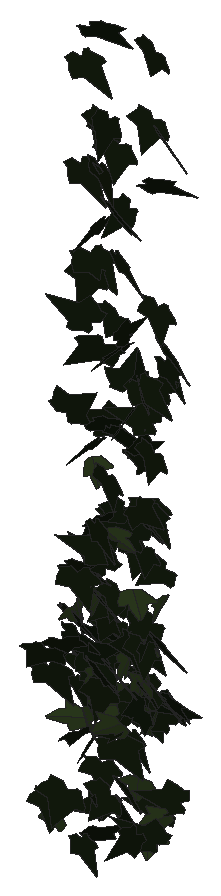
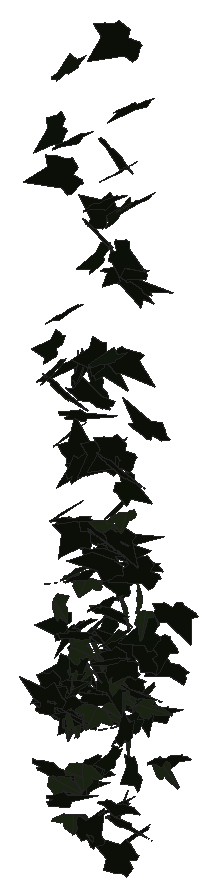
# SketchUp Ruby script. Lengths in inches.
U = 1.inch
M = Sketchup.active_model
def pt(a) = Geom::Point3d.new(a.map { |v| v * U })
def face(e, loops, mat)
  f = e.add_face(loops[0].map { |a| pt(a) })
  loops[1..].each { |l| e.add_face(l.map { |a| pt(a) }).erase! }
  f.material = f.back_material = mat if mat
  f
end
# faces: each face lists its corners as indices into pts; further lists are holes
def faces(e, pts, list, mat = nil) = list.each { |f| face(e, (f[0].is_a?(Array) ? f : [f]).map { |l| l.map { |i| pts[i] } }, mat) }
# xy, xz, yz: faces in a plane at the given z, y or x. An outline is a flat list of corners, or four numbers for a rectangle; further outlines are holes
def ring(l) = l.size == 4 ? [[l[0], l[1]], [l[2], l[1]], [l[2], l[3]], [l[0], l[3]]] : l.each_slice(2).to_a
def flat(e, list, mat, &to3) = list.each { |f| face(e, (f[0].is_a?(Array) ? f : [f]).map { |l| ring(l).map { |u, v| to3.(u, v) } }, mat) }
def xy(e, z, list, mat = nil) = flat(e, list, mat) { |x, y| [x, y, z] }
def xz(e, y, list, mat = nil) = flat(e, list, mat) { |x, z| [x, y, z] }
def yz(e, x, list, mat = nil) = flat(e, list, mat) { |y, z| [x, y, z] }
def lines(e, pts, list) = list.each { |a, b| e.add_line(pt(pts[a]), pt(pts[b])) }
# prism: a flat outline (further loops are holes) pulled along v
def prism(e, loops, v, mat = nil)
  f = face(e, loops, mat); d = Geom::Vector3d.new(v.map { |x| x * U })
  f.pushpull(f.normal.samedirection?(d) ? d.length : -d.length)
end
def box(e, o, s, mat = nil) = prism(e, [[o, [o[0] + s[0], o[1], o[2]], [o[0] + s[0], o[1] + s[1], o[2]], [o[0], o[1] + s[1], o[2]]]], [0, 0, s[2]], mat)
def at(x, y, z, deg = 0) = Geom::Transformation.translation(pt([x, y, z])) * Geom::Transformation.rotation(ORIGIN, Z_AXIS, deg.degrees)
def axes(o, x, y, z) = Geom::Transformation.new([*x, 0, *y, 0, *z, 0, *pt(o).to_a, 1])
def part(name) = M.definitions.add(name)
# library, detail: a bought-in or finely detailed component or shape, given as its bounding box
def library(name, o, s) = part(name).tap { |d| box(d.entities, o, s) }
def detail(e, o, s) = box(e.add_group.entities, o, s)
def put(e, d, t, mat = nil) = e.add_instance(d, t).tap { |i| i.material = mat if mat }
def group(e, t, mat = nil) = e.add_group.tap { |g| g.transformation = t; g.material = mat if mat }.entities
root = M.entities
M.materials.add("1026 AP 7946 SUNNY SIDE UP").color = [254, 231, 186]
M.materials.add("efeu1").color = [18, 25, 13]
M.materials.add("efeu2").color = [43, 57, 29]
c1 = part("ivyleaf_10")
p = [[0,0.5,-0.03],[-0.0625,2.02,-0.43],[-0.19,2.01,-0.46],[-0.54,1.05,-0.29],[-0.52,0.625,-0.18],[-0.83,0.76,-0.28],
  [-1.16,0.64,-0.33],[-1.15,0.33,-0.24],[-0.77,-0.39,0.02],[-0.3,-0.51,0.16],[0.04,-0.48,0.23],[-0.02,2.01,-0.4375],
  [-0.06,2.01,-0.43],[0.04,-0.49,0.23],[0.67,-0.49,0.14],[1.38,0.36,-0.2],[1.375,0.51,-0.24],[0.81,0.65,-0.19],
  [0.62,0.59,-0.15],[0.6,1.09,-0.28],[0.5,1.23,-0.31]]
faces(c1.entities,p,[[0,1,2,3,4,5,6,7,8,9,10],[11,12,0,13,14,15,16,17,18,19,20]],"efeu2")
c2 = part("ivyleaf_9")
p = [[1.54,2.16,1.25],[1.36,2.04,1.19],[-0.21,0.99,0.68],[-0.71,1.11,0.82],[-0.85,0.86,0.67],[-0.8,0.17,0.21],
  [-0.9,-0.01,0.1],[-0.67,-0.16,-0.02],[-0.08,-0.08,-0.05],[-0.03,-0.6,-0.4],[0.65,-0.88,-0.66],[0.83,-0.6,-0.49],
  [1.29,-0.42,-0.43],[1.8125,-0.07,-0.26],[1.21,0.44,0.15]]
faces(c2.entities,p,[[0,1,2,3,4,5,6,7,8,9,10,11,12,13,14]],"efeu1")
put(root,c1,axes([151.58,211.52,295.96],[-0.20274,0.31715,0.15198],[-0.2223,0.09458,-0.34036],[-0.50177,-0.17004,0.08938]),"1026 AP 7946 SUNNY SIDE UP")
put(root,c1,axes([151.39,211.94,305.0625],[0.21648,0.37675,-0.00006],[0.00323,-0.00309,-0.41323],[-0.5924,0.13765,-0.00227]),"1026 AP 7946 SUNNY SIDE UP")
put(root,c2,axes([151.69,211.69,306.17],[-0.31531,0.15411,-0.33038],[0.1841,-0.32003,-0.23508],[-0.52963,-0.20299,0.11498]),"1026 AP 7946 SUNNY SIDE UP")
put(root,c2,axes([151.3,212.07,296.14],[-0.06397,-0.10036,0.40641],[0.09147,-0.3944,-0.09935],[0.63438,0.04675,0.0553]),"1026 AP 7946 SUNNY SIDE UP")
put(root,c2,axes([151.6,209.85,299.05],[0.30367,0.3247,-0.13487],[-0.07387,-0.12624,-0.38923],[-0.54662,0.19744,-0.02232]),"1026 AP 7946 SUNNY SIDE UP")
put(root,c2,axes([152.11,211.9375,306.89],[-0.32903,0.23875,0.28411],[-0.36666,0.15494,-0.32113],[-0.43898,-0.30837,0.05528]),"1026 AP 7946 SUNNY SIDE UP")
put(root,c2,axes([152.14,211.23,297.44],[-0.29031,0.18556,0.30476],[-0.50067,0.04533,-0.23459],[-0.22203,-0.34485,0.13052]),"1026 AP 7946 SUNNY SIDE UP")
put(root,c2,axes([151.23,210.59,299.79],[0.61515,-0.18915,0.06263],[0.06028,-0.06227,-0.44622],[0.30706,0.39115,-0.03787]),"1026 AP 7946 SUNNY SIDE UP")
put(root,c2,axes([151.68,210.97,294.125],[0.07882,0.17846,0.39297],[0.17368,0.36407,-0.1888],[-0.63752,0.12125,-0.00285]),"1026 AP 7946 SUNNY SIDE UP")
put(root,c2,axes([151.33,209.54,298.03],[-0.23555,-0.13651,-0.39631],[0.50676,0.2106,-0.20546],[0.39205,-0.35424,0.02746]),"1026 AP 7946 SUNNY SIDE UP")
put(root,c2,axes([151.37,210.48,307.77],[-0.25898,0.1451,0.40132],[0.48152,-0.23971,0.22444],[0.44026,0.34754,-0.0094]),"1026 AP 7946 SUNNY SIDE UP")
put(root,c2,axes([151.18,210.74,298.82],[0.2905,-0.06507,-0.36411],[0.55995,0.08361,0.17658],[0.07165,-0.38961,0.09626]),"1026 AP 7946 SUNNY SIDE UP")
put(root,c1,axes([151.73,210.37,300.15],[-0.15359,-0.35607,-0.15589],[0.08392,0.14008,-0.37931],[0.60129,-0.1105,0.01312]),"1026 AP 7946 SUNNY SIDE UP")
put(root,c2,axes([151.41,211.29,321.42],[0.17929,-0.39421,-0.24325],[0.04295,0.24643,-0.41274],[0.71947,0.08353,0.08526]),"1026 AP 7946 SUNNY SIDE UP")
put(root,c2,axes([151.59,211.0625,296.29],[0.51591,-0.10317,-0.20405],[-0.23838,0.15422,-0.34159],[0.25673,0.35052,0.09286]),"1026 AP 7946 SUNNY SIDE UP")
put(root,c2,axes([151.53,210.72,297.15],[0.14112,-0.37276,0.1134],[0.05437,-0.10705,-0.39553],[0.60968,0.09583,0.00902]),"1026 AP 7946 SUNNY SIDE UP")
put(root,c2,axes([152.04,208.41,299.49],[0.23818,0.21822,-0.31605],[-0.2899,-0.24685,-0.27501],[-0.51796,0.23851,0.00859]),"1026 AP 7946 SUNNY SIDE UP")
put(root,c1,axes([152.23,209.99,296.18],[-0.17607,0.0833,0.38101],[-0.45487,-0.26734,-0.0298],[0.38414,-0.27839,0.13934]),"1026 AP 7946 SUNNY SIDE UP")
put(root,c2,axes([151.7,211.98,293.24],[-0.32935,-0.24898,-0.17657],[0.25381,0.08219,-0.32845],[0.40037,-0.25693,0.06297]),"1026 AP 7946 SUNNY SIDE UP")
put(root,c2,axes([151.56,211.02,317.34],[0.1728,-0.4241,-0.1714],[0.01793,0.17121,-0.44732],[0.71474,0.09824,0.05266]),"1026 AP 7946 SUNNY SIDE UP")
put(root,c1,axes([151.97,211.76,297.97],[0.01802,-0.32103,0.23921],[-0.00152,-0.23414,-0.33221],[0.62467,0.00869,-0.00771]),"1026 AP 7946 SUNNY SIDE UP")
put(root,c2,axes([151.74,211.48,298.84],[0.6021,0.09468,-0.06166],[-0.07701,-0.05233,-0.40471],[-0.1589,0.3841,-0.03751]),"1026 AP 7946 SUNNY SIDE UP")
put(root,c2,axes([152.33,211.37,292.15],[-0.53213,0.07532,0.13666],[-0.21747,-0.01774,-0.35435],[-0.09981,-0.3629,0.04347]),"1026 AP 7946 SUNNY SIDE UP")
put(root,c2,axes([151.84,211.97,318.77],[-0.17635,-0.39075,0.18902],[-0.02111,-0.1886,-0.41829],[0.67994,-0.1072,0.03604]),"1026 AP 7946 SUNNY SIDE UP")
put(root,c2,axes([152.19,211.78,298.01],[-0.09194,0.39723,-0.02018],[-0.00777,-0.02281,-0.41368],[-0.62549,-0.0581,0.00811]),"1026 AP 7946 SUNNY SIDE UP")
put(root,c1,axes([152.01,211.31,297.37],[0.02087,-0.29789,0.26728],[0.03755,-0.2602,-0.30857],[0.62177,0.02571,0.00966]),"1026 AP 7946 SUNNY SIDE UP")
put(root,c2,axes([151.91,211.88,296.28],[-0.28748,-0.32289,0.11068],[0.07705,-0.1476,-0.36573],[0.53043,-0.15356,0.11311]),"1026 AP 7946 SUNNY SIDE UP")
put(root,c2,axes([151.75,212.14,295.1],[0.33403,-0.30879,0.07536],[0.0319,-0.07674,-0.38562],[0.4986,0.21178,-0.02582]),"1026 AP 7946 SUNNY SIDE UP")
put(root,c2,axes([151.8,211.73,317.04],[0.19243,-0.41509,0.12377],[0.01909,-0.12396,-0.44594],[0.68025,0.1209,-0.0225]),"1026 AP 7946 SUNNY SIDE UP")
put(root,c2,axes([152.23,211.3,315.1875],[-0.28394,0.14182,-0.38811],[0.27614,-0.34473,-0.22195],[-0.57087,-0.23729,0.08567]),"1026 AP 7946 SUNNY SIDE UP")
put(root,c1,axes([152.54,208.48,293.02],[-0.28676,0.10932,0.34754],[-0.54081,0.03509,-0.20343],[-0.13198,-0.38133,0.07847]),"1026 AP 7946 SUNNY SIDE UP")
put(root,c2,axes([151.74,211.39,290.74],[0.36507,0.33301,-0.12852],[0.07542,0.12057,0.4179],[0.55511,-0.23538,0.02775]),"1026 AP 7946 SUNNY SIDE UP")
put(root,c2,axes([151.75,210.17,301.92],[0.55829,0.08731,0.16743],[0.26095,0.00034,-0.37485],[-0.12512,0.39028,-0.03473]),"1026 AP 7946 SUNNY SIDE UP")
put(root,c2,axes([152.34,211.125,303.61],[-0.10982,0.32752,-0.22879],[0.06296,-0.22041,-0.34623],[-0.62069,-0.08031,0.00536]),"1026 AP 7946 SUNNY SIDE UP")
put(root,c2,axes([152.17,212.08,298.95],[-0.3055,-0.32778,0.05232],[0.03482,-0.07366,-0.38869],[0.52084,-0.18734,0.05667]),"1026 AP 7946 SUNNY SIDE UP")
put(root,c2,axes([152.12,208.7,293.53],[-0.25278,-0.36459,-0.05549],[0.05155,0.04212,-0.41003],[0.57674,-0.16356,0.01233]),"1026 AP 7946 SUNNY SIDE UP")
put(root,c2,axes([152.1,212.37,317.6875],[-0.192,-0.43373,0.05883],[0.00137,-0.06208,-0.46421],[0.6884,-0.12085,0.01733]),"1026 AP 7946 SUNNY SIDE UP")
put(root,c2,axes([151.95,211.26,297.97],[-0.16724,-0.25735,-0.32678],[0.27957,0.26427,-0.28206],[0.57625,-0.2029,0.042]),"1026 AP 7946 SUNNY SIDE UP")
put(root,c2,axes([152.57,210.9,310.63],[0.06854,0.11936,-0.45955],[-0.24261,-0.41927,-0.13336],[-0.68546,0.16033,0.00125]),"1026 AP 7946 SUNNY SIDE UP")
put(root,c2,axes([151.98,211.33,307.18],[0.54069,0.22505,0.1565],[0.21127,0.06962,-0.4227],[-0.36972,0.3689,-0.01267]),"1026 AP 7946 SUNNY SIDE UP")
put(root,c2,axes([152.3,210.66,313.57],[-0.62889,-0.07015,-0.22927],[0.35265,0.00344,-0.41708],[0.09909,-0.4575,0.02928]),"1026 AP 7946 SUNNY SIDE UP")
put(root,c2,axes([152.25,211.24,292.16],[-0.11367,0.04227,0.37021],[-0.14164,-0.35679,0.02249],[0.55065,-0.08305,0.08221]),"1026 AP 7946 SUNNY SIDE UP")
put(root,c1,axes([152.41,210.77,300.6],[0.2429,-0.31779,-0.19028],[-0.11409,0.16805,-0.36296],[0.56515,0.17051,0.00851]),"1026 AP 7946 SUNNY SIDE UP")
put(root,c2,axes([152.22,212.18,311.08],[-0.31051,-0.30089,0.24499],[0.09344,-0.28989,-0.32638],[0.59746,-0.11104,0.17837]),"1026 AP 7946 SUNNY SIDE UP")
put(root,c1,axes([152.72,211.125,296.32],[0.22908,-0.06543,-0.35023],[-0.52536,0.06854,-0.16087],[0.14045,0.36312,-0.03048]),"1026 AP 7946 SUNNY SIDE UP")
put(root,c2,axes([152.19,210.26,291.16],[0.13155,-0.3686,-0.10444],[-0.03749,0.0964,-0.38882],[0.59908,0.08697,-0.0014]),"1026 AP 7946 SUNNY SIDE UP")
put(root,c1,axes([152.21,210.08,300.61],[-0.07812,0.13731,-0.38589],[0.18678,-0.35609,-0.15247],[-0.60008,-0.12871,0.00278]),"1026 AP 7946 SUNNY SIDE UP")
put(root,c2,axes([152.59,212.125,303.3],[-0.55104,-0.19549,0.03116],[-0.01456,-0.04749,-0.41192],[0.31097,-0.34862,0.03593]),"1026 AP 7946 SUNNY SIDE UP")
put(root,c2,axes([152.3,211.48,299.48],[-0.15496,-0.31275,0.23884],[0.03028,-0.24455,-0.33033],[0.61308,-0.06697,0.07668]),"1026 AP 7946 SUNNY SIDE UP")
put(root,c2,axes([152.48,211.39,292.56],[-0.28112,-0.33521,0.24878],[-0.11167,-0.23636,-0.39048],[0.64172,-0.18797,0.04103]),"1026 AP 7946 SUNNY SIDE UP")
put(root,c2,axes([152.17,211.7,302.85],[0.15089,0.23036,-0.37165],[0.05267,0.36585,0.25108],[0.67271,-0.08031,0.0637]),"1026 AP 7946 SUNNY SIDE UP")
put(root,c2,axes([152.65,211.85,303.71],[-0.59768,0.01456,-0.13021],[0.18641,-0.10475,-0.38006],[-0.073,-0.38666,0.09563]),"1026 AP 7946 SUNNY SIDE UP")
put(root,c2,axes([152.3,209.92,301.91],[-0.23219,-0.31547,-0.20929],[0.22344,0.15299,-0.3534],[0.54441,-0.19734,0.05579]),"1026 AP 7946 SUNNY SIDE UP")
put(root,c2,axes([152.6875,209.41,296.01],[0.05627,0.39325,-0.08438],[-0.00885,-0.08398,-0.40729],[-0.63229,0.03617,-0.00181]),"1026 AP 7946 SUNNY SIDE UP")
put(root,c2,axes([152.48,211.34,319.26],[-0.56202,-0.00418,-0.31958],[0.48512,-0.05422,-0.36581],[-0.05094,-0.47014,0.04224]),"1026 AP 7946 SUNNY SIDE UP")
put(root,c2,axes([153.03,210.39,302.82],[-0.26275,0.05031,0.41716],[-0.63006,-0.1013,-0.15808],[0.11882,-0.42591,0.08421]),"1026 AP 7946 SUNNY SIDE UP")
put(root,c2,axes([152.25,210.74,314.18],[-0.07528,-0.34773,-0.303],[0.20853,0.27026,-0.3522],[0.68301,-0.12084,0.07413]),"1026 AP 7946 SUNNY SIDE UP")
put(root,c2,axes([152.14,210.52,298.49],[0.02126,-0.04056,0.44097],[0.66151,-0.08829,-0.02281],[0.14135,0.4193,0.04044]),"1026 AP 7946 SUNNY SIDE UP")
put(root,c2,axes([153.12,210.29,302.35],[-0.01259,0.05145,0.45165],[-0.56202,0.25605,-0.03621],[-0.40651,-0.3556,0.03607]),"1026 AP 7946 SUNNY SIDE UP")
put(root,c2,axes([152.88,211.32,300.47],[-0.58184,-0.11464,0.02148],[-0.015,-0.04153,-0.39752],[0.18278,-0.36832,0.03575]),"1026 AP 7946 SUNNY SIDE UP")
put(root,c2,axes([152.96,211.85,298.17],[-0.54397,0.13185,-0.10086],[0.12546,-0.06657,-0.38031],[-0.2265,-0.35353,0.03156]),"1026 AP 7946 SUNNY SIDE UP")
put(root,c2,axes([153.33,209.21,312.63],[-0.20829,0.17221,0.39501],[-0.59091,0.12941,-0.19336],[-0.29293,-0.3835,0.10918]),"1026 AP 7946 SUNNY SIDE UP")
put(root,c2,axes([152.5,211.57,306.96],[0.66442,0.03779,-0.01428],[-0.01623,-0.04186,-0.43527],[-0.0613,0.42071,-0.03952]),"1026 AP 7946 SUNNY SIDE UP")
put(root,c1,axes([152.76,211.96,296.65],[-0.5574,-0.10251,-0.09313],[0.1571,-0.02521,-0.37672],[0.14576,-0.36482,0.04989]),"1026 AP 7946 SUNNY SIDE UP")
put(root,c2,axes([152.49,210.5,323.37],[0.65377,0.19814,0.12409],[0.19189,0.0206,-0.47316],[-0.30896,0.43207,-0.03128]),"1026 AP 7946 SUNNY SIDE UP")
put(root,c2,axes([153.11,211.22,310.52],[-0.26407,0.30804,-0.2652],[0.0734,-0.26403,-0.35599],[-0.62872,-0.16021,0.06982]),"1026 AP 7946 SUNNY SIDE UP")
put(root,c2,axes([152.5,210.41,301.15],[0.38272,-0.27949,0.19652],[0.16758,-0.16177,-0.38202],[0.50649,0.26472,-0.02211]),"1026 AP 7946 SUNNY SIDE UP")
put(root,c2,axes([152.89,211.39,300.73],[-0.18925,-0.3553,0.10281],[-0.03567,-0.09978,-0.38691],[0.58007,-0.12206,0.00975]),"1026 AP 7946 SUNNY SIDE UP")
put(root,c2,axes([153.15,211.57,315.93],[-0.63558,0.09146,-0.16879],[0.24003,-0.0681,-0.42619],[-0.17279,-0.431,0.02883]),"1026 AP 7946 SUNNY SIDE UP")
put(root,c1,axes([152.79,209.75,296.6],[-0.25188,0.2073,-0.3118],[0.22002,-0.27214,-0.26887],[-0.53488,-0.20957,0.03623]),"1026 AP 7946 SUNNY SIDE UP")
put(root,c2,axes([152.88,211.5,310.75],[0.06501,0.11253,0.44745],[0.40104,0.35218,-0.11713],[-0.57925,0.25646,-0.03088]),"1026 AP 7946 SUNNY SIDE UP")
put(root,c2,axes([153.17,211.76,291.3125],[0.36801,-0.25612,0.26277],[-0.19021,0.23266,0.35436],[-0.53731,-0.25778,0.05453]),"1026 AP 7946 SUNNY SIDE UP")
put(root,c2,axes([153.34,211.66,296.21],[-0.52005,-0.17464,0.1455],[-0.1717,-0.09667,-0.38443],[0.30975,-0.3468,0.03119]),"1026 AP 7946 SUNNY SIDE UP")
put(root,c2,axes([153.25,211.61,308.96],[-0.61027,0.07069,0.19717],[0.29407,-0.03901,0.40616],[0.12677,0.4308,0.00703]),"1026 AP 7946 SUNNY SIDE UP")
put(root,c2,axes([152.79,210.24,298.11],[0.26743,-0.20976,0.29945],[0.22377,-0.2572,-0.27737],[0.51897,0.21899,-0.03471]),"1026 AP 7946 SUNNY SIDE UP")
put(root,c2,axes([153.16,212.25,302.18],[-0.18872,-0.36471,0.07998],[-0.02888,-0.07785,-0.39593],[0.58629,-0.12123,0.00624]),"1026 AP 7946 SUNNY SIDE UP")
put(root,c1,axes([153.31,212.29,299.1],[-0.11247,-0.20951,0.34739],[0.00842,-0.3443,-0.22045],[0.62577,-0.03303,0.0654]),"1026 AP 7946 SUNNY SIDE UP")
put(root,c2,axes([153.86,211.22,303.23],[-0.32049,0.11701,0.38166],[-0.55481,0.11759,-0.23798],[-0.25333,-0.40556,0.03835]),"1026 AP 7946 SUNNY SIDE UP")
put(root,c1,axes([153.08,210.74,303.4],[-0.42269,-0.11238,-0.28786],[0.42969,0.06443,-0.29783],[0.19689,-0.38188,0.03197]),"1026 AP 7946 SUNNY SIDE UP")
put(root,c2,axes([153.1,209.91,304.07],[0.2978,-0.37235,-0.08131],[-0.09,0.05691,-0.42927],[0.59099,0.19629,-0.0244]),"1026 AP 7946 SUNNY SIDE UP")
put(root,c2,axes([153.4,207.87,294.58],[-0.37427,-0.39701,0.04747],[-0.00778,-0.05331,-0.47659],[0.62882,-0.23695,0.02235]),"1026 AP 7946 SUNNY SIDE UP")
put(root,c2,axes([153.38,209.9375,297.75],[-0.51748,-0.10914,-0.23059],[0.36516,-0.0034,-0.35104],[0.13891,-0.39764,0.06379]),"1026 AP 7946 SUNNY SIDE UP")
put(root,c2,axes([153.33,212.31,302.21],[-0.08847,-0.35835,0.15348],[0.06025,-0.15696,-0.3699],[0.60848,-0.03656,0.05894]),"1026 AP 7946 SUNNY SIDE UP")
put(root,c2,axes([153.47,212.06,298.22],[-0.23921,0.01876,0.37048],[0.02773,-0.38944,0.02635],[0.5654,0.02704,0.15545]),"1026 AP 7946 SUNNY SIDE UP")
put(root,c2,axes([153.63,212.07,306.01],[-0.00544,0.00956,0.46455],[-0.38987,-0.37667,0.00406],[0.59233,-0.24784,0.00694]),"1026 AP 7946 SUNNY SIDE UP")
put(root,c2,axes([153.76,212.1,299.5],[-0.50414,-0.19645,0.11636],[-0.1064,-0.10576,-0.3842],[0.34097,-0.32345,0.05216]),"1026 AP 7946 SUNNY SIDE UP")
put(root,c1,axes([153.64,210.83,298.47],[0.37945,-0.31512,-0.08102],[-0.05911,0.06797,-0.40833],[0.50658,0.24397,0.01304]),"1026 AP 7946 SUNNY SIDE UP")
put(root,c2,axes([153.67,211.19,292.95],[0.24683,-0.36967,0.07199],[-0.01132,0.07502,0.41354],[-0.59208,-0.15555,0.0221]),"1026 AP 7946 SUNNY SIDE UP")
put(root,c1,axes([153.72,212.07,296.17],[0.02246,-0.37033,0.04496],[-0.00545,-0.04591,-0.38203],[0.58671,0.01375,-0.00527]),"1026 AP 7946 SUNNY SIDE UP")
put(root,c2,axes([153.49,211.9375,303.68],[0.61626,0.05162,-0.09495],[-0.13644,-0.0466,-0.40601],[-0.09544,0.39998,-0.03264]),"1026 AP 7946 SUNNY SIDE UP")
put(root,c2,axes([153.17,210.85,316.07],[0.21303,-0.27348,0.37446],[0.30878,-0.30873,-0.31517],[0.64733,0.23726,0.0271]),"1026 AP 7946 SUNNY SIDE UP")
put(root,c2,axes([153.43,211.91,297.34],[0.08165,-0.35334,0.16077],[0.05369,-0.15467,-0.36867],[0.60628,0.06128,0.011]),"1026 AP 7946 SUNNY SIDE UP")
put(root,c2,axes([153.35,210.82,314.38],[0.43069,-0.36529,-0.00659],[-0.03185,-0.0098,-0.46987],[0.57354,0.27376,-0.02114]),"1026 AP 7946 SUNNY SIDE UP")
put(root,c2,axes([153.45,210.125,306.05],[0.05493,-0.40863,0.18548],[0.03048,-0.18137,-0.42355],[0.70295,0.0398,0.00387]),"1026 AP 7946 SUNNY SIDE UP")
put(root,c2,axes([154.23,211.45,307.9],[-0.35346,0.10615,0.33959],[-0.5371,-0.12886,-0.19833],[0.08404,-0.37708,0.16073]),"1026 AP 7946 SUNNY SIDE UP")
put(root,c2,axes([153.54,211.97,296.18],[-0.18684,-0.25399,-0.30476],[0.21189,0.26184,-0.28724],[0.57348,-0.1795,0.00684]),"1026 AP 7946 SUNNY SIDE UP")
put(root,c1,axes([153.89,211.28,293.62],[-0.5485,-0.12629,0.04339],[-0.04224,-0.05095,-0.38042],[0.20539,-0.34774,0.03764]),"1026 AP 7946 SUNNY SIDE UP")
put(root,c2,axes([154.16,211.77,297.13],[-0.54019,-0.12066,0.25135],[-0.33569,-0.12602,-0.37358],[0.26704,-0.4025,0.03883]),"1026 AP 7946 SUNNY SIDE UP")
put(root,c1,axes([154.11,211.19,297.6],[-0.47399,0.09137,0.21738],[-0.3445,-0.01131,-0.31825],[-0.10724,-0.36748,0.06156]),"1026 AP 7946 SUNNY SIDE UP")
put(root,c2,axes([153.86,211.19,298.9],[0.21677,-0.39718,-0.19],[0.11039,-0.16841,0.43201],[-0.67816,-0.15437,0.00959]),"1026 AP 7946 SUNNY SIDE UP")
put(root,c2,axes([153.73,211.5,306.53],[0.40154,0.2509,0.24251],[-0.3109,-0.13073,0.36596],[0.44083,-0.32073,0.0372]),"1026 AP 7946 SUNNY SIDE UP")
put(root,c2,axes([153.85,212.08,319.45],[-0.23101,-0.40291,0.13821],[-0.03588,-0.13668,-0.44191],[0.66792,-0.1467,0.02406]),"1026 AP 7946 SUNNY SIDE UP")
put(root,c2,axes([153.68,212.06,304.19],[-0.11816,-0.37689,-0.13538],[0.2103,0.10005,-0.38004],[0.59016,-0.11112,0.10832]),"1026 AP 7946 SUNNY SIDE UP")
put(root,c2,axes([154.08,212.41,301.61],[-0.45566,-0.19719,0.18896],[-0.07173,-0.23105,-0.32948],[0.41857,-0.25426,0.14925]),"1026 AP 7946 SUNNY SIDE UP")
put(root,c2,axes([153.58,209.97,298.69],[0.49088,-0.24853,0.0644],[0.05225,-0.06068,-0.41054],[0.40012,0.31283,-0.02541]),"1026 AP 7946 SUNNY SIDE UP")
put(root,c2,axes([153.71,211.15,295.46],[0.24596,-0.37486,-0.00374],[-0.01627,-0.00269,-0.41833],[0.58921,0.15641,-0.00999]),"1026 AP 7946 SUNNY SIDE UP")
put(root,c1,axes([154.03,211.45,297.7],[0.0951,-0.32164,-0.23941],[0.0509,0.23648,-0.32972],[0.62018,0.02991,0.06377]),"1026 AP 7946 SUNNY SIDE UP")
put(root,c1,axes([154.07,211.8,295.89],[-0.01452,-0.37423,-0.11978],[0.03271,0.11354,-0.38457],[0.61432,-0.01489,0.01764]),"1026 AP 7946 SUNNY SIDE UP")
put(root,c2,axes([154.11,211.09,309.47],[-0.07286,-0.31266,0.30146],[0.26765,0.25849,0.31192],[-0.61996,0.14834,0.09923]),"1026 AP 7946 SUNNY SIDE UP")
put(root,c2,axes([153.54,211.95,296.26],[0.38917,-0.02405,0.33125],[0.48393,-0.10385,-0.25255],[0.15194,0.39236,-0.04408]),"1026 AP 7946 SUNNY SIDE UP")
put(root,c2,axes([154.58,211.93,295.94],[-0.17643,0.12668,0.37107],[-0.48253,0.19221,-0.16734],[-0.35542,-0.32383,0.04299]),"1026 AP 7946 SUNNY SIDE UP")
put(root,c1,axes([153.91,211.46,298.93],[0.57744,-0.05861,0.11728],[0.17318,-0.03376,-0.38299],[0.1036,0.38309,-0.0135]),"1026 AP 7946 SUNNY SIDE UP")
put(root,c1,axes([153.91,210.98,301.12],[0.51195,0.19408,0.10072],[0.1284,0.0518,-0.39017],[-0.31582,0.33566,0.00464]),"1026 AP 7946 SUNNY SIDE UP")
put(root,c1,axes([154.53,209.21,297.01],[-0.3998,-0.08793,0.31046],[-0.42401,-0.13862,-0.27641],[0.2542,-0.36953,0.02723]),"1026 AP 7946 SUNNY SIDE UP")
put(root,c2,axes([153.95,212.08,322.2],[-0.14272,-0.32537,0.32994],[0.06636,-0.33293,-0.33615],[0.71686,-0.03396,0.09681]),"1026 AP 7946 SUNNY SIDE UP")
put(root,c2,axes([154.18,209.82,308.33],[0.12843,0.18063,0.43616],[0.1878,0.40587,-0.20024],[-0.69745,0.14255,0.0264]),"1026 AP 7946 SUNNY SIDE UP")
put(root,c2,axes([154.57,211.93,292.44],[-0.20489,-0.29322,-0.24465],[-0.16274,-0.212,0.32924],[-0.56884,0.16627,-0.00607]),"1026 AP 7946 SUNNY SIDE UP")
put(root,c2,axes([154.72,211.79,309.1],[-0.34147,0.22763,0.28376],[-0.32996,0.17778,-0.32228],[-0.45285,-0.30119,0.02085]),"1026 AP 7946 SUNNY SIDE UP")
put(root,c1,axes([154.27,212.16,300.5625],[0.06254,-0.36004,0.16811],[0.04973,-0.16264,-0.3739],[0.62091,0.04929,0.01301]),"1026 AP 7946 SUNNY SIDE UP")
put(root,c2,axes([154.14,211.44,297.2],[0.3927,-0.31179,-0.0806],[0.11464,-0.03926,0.41001],[-0.49159,-0.25822,0.03123]),"1026 AP 7946 SUNNY SIDE UP")
put(root,c1,axes([154.17,211.37,291.58],[0.45323,0.27179,-0.01186],[0.01301,-0.02776,-0.40742],[-0.42765,0.28719,-0.02496]),"1026 AP 7946 SUNNY SIDE UP")
put(root,c2,axes([154.64,209.39,296.81],[-0.32746,0.36084,0.02663],[-0.05695,0.00651,-0.42819],[-0.56576,-0.20951,0.02769]),"1026 AP 7946 SUNNY SIDE UP")
put(root,c2,axes([154.22,211.14,299.22],[-0.10546,-0.40863,0.03132],[0.00044,-0.03321,-0.42676],[0.64459,-0.06683,0.00542]),"1026 AP 7946 SUNNY SIDE UP")
put(root,c2,axes([154.12,211.72,304.26],[0.15189,-0.39483,-0.08509],[0.00467,0.08333,-0.41763],[0.63354,0.09404,0.02348]),"1026 AP 7946 SUNNY SIDE UP")
put(root,c2,axes([154.29,211.23,299.16],[0.21258,-0.26457,-0.31894],[-0.26002,0.26071,-0.30387],[0.58321,0.21267,-0.01922]),"1026 AP 7946 SUNNY SIDE UP")
put(root,c2,axes([154.22,211.91,312.24],[-0.04713,-0.43959,0.05102],[0.00233,-0.05224,-0.45419],[0.69603,-0.02959,0.00497]),"1026 AP 7946 SUNNY SIDE UP")
put(root,c2,axes([154.1,209.84,295.91],[-0.1166,-0.29848,-0.32496],[0.30133,0.26282,-0.30271],[0.6106,-0.1867,0.08733]),"1026 AP 7946 SUNNY SIDE UP")
put(root,c2,axes([154.25,211.09,309.14],[-0.01685,-0.08972,0.43061],[-0.00705,-0.41858,-0.09502],[0.67296,-0.00663,0.00979]),"1026 AP 7946 SUNNY SIDE UP")
put(root,c2,axes([155.07,210.0625,297.42],[0.09349,-0.04788,-0.47321],[-0.72546,0.00683,-0.06226],[0.02037,0.46285,-0.04529]),"1026 AP 7946 SUNNY SIDE UP")
put(root,c2,axes([154.42,212.15,309.96],[0.2569,-0.39533,-0.02203],[-0.038,0.01071,-0.44022],[0.62119,0.16415,-0.01782]),"1026 AP 7946 SUNNY SIDE UP")
put(root,c2,axes([154.4,210.77,309.78],[0.19081,-0.33683,-0.2883],[0.0209,0.29119,-0.35586],[0.68635,0.08478,0.09098]),"1026 AP 7946 SUNNY SIDE UP")
put(root,c2,axes([154.55,211.27,306.85],[-0.08456,-0.3747,0.22176],[-0.01973,-0.21762,-0.39089],[0.68087,-0.05284,0.01622]),"1026 AP 7946 SUNNY SIDE UP")
put(root,c2,axes([155.23,210.44,292.08],[-0.10983,0.08367,0.42663],[-0.66115,0.02223,-0.07764],[-0.05703,-0.41892,0.07854]),"1026 AP 7946 SUNNY SIDE UP")
put(root,c1,axes([155.03,211.19,292.7],[-0.21076,-0.15228,0.33095],[-0.26026,-0.27815,-0.20805],[0.49612,-0.2106,0.03145]),"1026 AP 7946 SUNNY SIDE UP")
put(root,c2,axes([154.5625,211.8,297.01],[0.59303,-0.03482,-0.01833],[-0.03249,-0.03322,-0.38872],[0.05204,0.37609,-0.03379]),"1026 AP 7946 SUNNY SIDE UP")
put(root,c2,axes([154.71,210.18,305.26],[0.11127,-0.15996,-0.38286],[-0.13843,0.36121,-0.17576],[0.6196,0.10943,0.02949]),"1026 AP 7946 SUNNY SIDE UP")
put(root,c2,axes([154.44,211.22,317.5],[0.57612,0.09235,0.24962],[0.35286,0.09542,-0.38733],[-0.20275,0.42848,0.0352]),"1026 AP 7946 SUNNY SIDE UP")
put(root,c2,axes([154.5,211.41,297.45],[0.42628,-0.26969,0.10159],[0.07771,-0.0919,-0.39332],[0.44563,0.27401,-0.02859]),"1026 AP 7946 SUNNY SIDE UP")
put(root,c2,axes([154.9375,209.71,292.55],[-0.06074,-0.04027,-0.46509],[0.26611,-0.42137,0.02135],[-0.66077,-0.16599,0.05135]),"1026 AP 7946 SUNNY SIDE UP")
put(root,c2,axes([154.49,211.48,299.32],[0.45165,-0.21762,0.15389],[0.15399,-0.11909,-0.37038],[0.38661,0.30167,-0.03225]),"1026 AP 7946 SUNNY SIDE UP")
put(root,c2,axes([155.43,211.52,293.25],[-0.39446,0.09206,0.30683],[-0.47715,0.01256,-0.26771],[-0.10881,-0.38881,0.06159]),"1026 AP 7946 SUNNY SIDE UP")
put(root,c2,axes([154.55,211.93,310.73],[0.36465,-0.33795,0.12912],[0.08207,-0.11828,-0.42227],[0.56185,0.23661,-0.02212]),"1026 AP 7946 SUNNY SIDE UP")
put(root,c2,axes([154.46,212.2,296.4],[0.14306,-0.08411,0.42611],[0.44199,-0.30422,-0.12906],[0.49608,0.2953,-0.00789]),"1026 AP 7946 SUNNY SIDE UP")
put(root,c2,axes([154.7,211.47,319.42],[0.60979,-0.23701,-0.13788],[-0.19932,0.04625,-0.46721],[0.37756,0.4072,-0.02396]),"1026 AP 7946 SUNNY SIDE UP")
